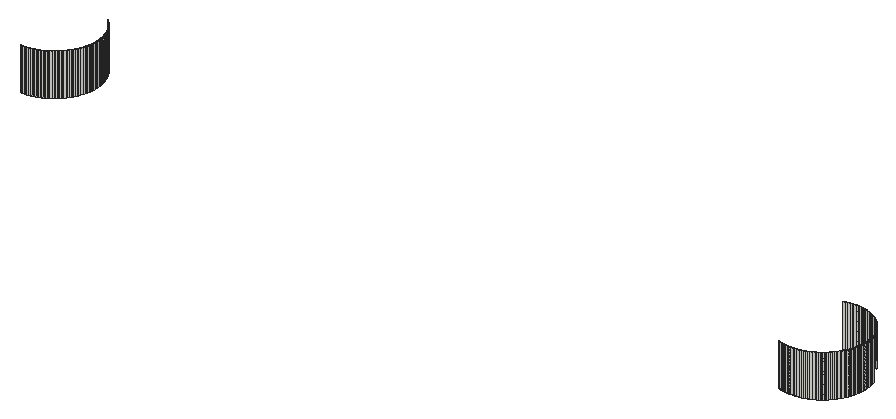
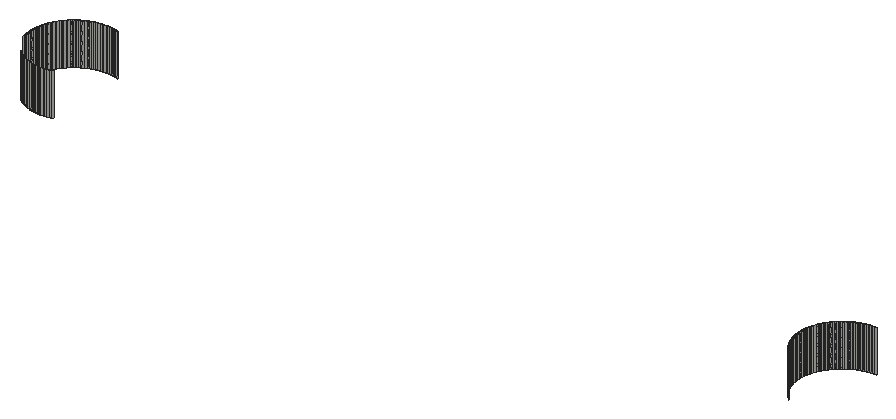
# SketchUp Ruby script. Lengths in inches.
U = 1.inch
M = Sketchup.active_model
def pt(a) = Geom::Point3d.new(a.map { |v| v * U })
def face(e, loops, mat)
  f = e.add_face(loops[0].map { |a| pt(a) })
  loops[1..].each { |l| e.add_face(l.map { |a| pt(a) }).erase! }
  f.material = f.back_material = mat if mat
  f
end
# faces: each face lists its corners as indices into pts; further lists are holes
def faces(e, pts, list, mat = nil) = list.each { |f| face(e, (f[0].is_a?(Array) ? f : [f]).map { |l| l.map { |i| pts[i] } }, mat) }
# xy, xz, yz: faces in a plane at the given z, y or x. An outline is a flat list of corners, or four numbers for a rectangle; further outlines are holes
def ring(l) = l.size == 4 ? [[l[0], l[1]], [l[2], l[1]], [l[2], l[3]], [l[0], l[3]]] : l.each_slice(2).to_a
def flat(e, list, mat, &to3) = list.each { |f| face(e, (f[0].is_a?(Array) ? f : [f]).map { |l| ring(l).map { |u, v| to3.(u, v) } }, mat) }
def xy(e, z, list, mat = nil) = flat(e, list, mat) { |x, y| [x, y, z] }
def xz(e, y, list, mat = nil) = flat(e, list, mat) { |x, z| [x, y, z] }
def yz(e, x, list, mat = nil) = flat(e, list, mat) { |y, z| [x, y, z] }
def lines(e, pts, list) = list.each { |a, b| e.add_line(pt(pts[a]), pt(pts[b])) }
# prism: a flat outline (further loops are holes) pulled along v
def prism(e, loops, v, mat = nil)
  f = face(e, loops, mat); d = Geom::Vector3d.new(v.map { |x| x * U })
  f.pushpull(f.normal.samedirection?(d) ? d.length : -d.length)
end
def box(e, o, s, mat = nil) = prism(e, [[o, [o[0] + s[0], o[1], o[2]], [o[0] + s[0], o[1] + s[1], o[2]], [o[0], o[1] + s[1], o[2]]]], [0, 0, s[2]], mat)
def at(x, y, z, deg = 0) = Geom::Transformation.translation(pt([x, y, z])) * Geom::Transformation.rotation(ORIGIN, Z_AXIS, deg.degrees)
def axes(o, x, y, z) = Geom::Transformation.new([*x, 0, *y, 0, *z, 0, *pt(o).to_a, 1])
def part(name) = M.definitions.add(name)
# library, detail: a bought-in or finely detailed component or shape, given as its bounding box
def library(name, o, s) = part(name).tap { |d| box(d.entities, o, s) }
def detail(e, o, s) = box(e.add_group.entities, o, s)
def put(e, d, t, mat = nil) = e.add_instance(d, t).tap { |i| i.material = mat if mat }
def group(e, t, mat = nil) = e.add_group.tap { |g| g.transformation = t; g.material = mat if mat }.entities
root = M.entities
xz(root,317,[[269.15,231,269.23,234],[269.23,231,269.3125,234],[323.875,231,323.95,234],[323.95,231,324.03,234],[324.03,231,324.11,234]])
xz(root,317.01,[[269.39,231,269.47,234],[323.72,231,323.8,234],[324.19,231,324.27,234]])
xz(root,322.99,[[323.73,231,323.81,234],[324.2,231,324.28,234]])
xz(root,323,[[323.89,231,323.97,234],[323.97,231,324.05,234],[324.05,231,324.125,234]])
yz(root,272.2,[[319.875,231,319.95,234],[319.95,231,320.03,234],[320.03,231,320.11,234]])
yz(root,326.99,[[319.72,231,319.8,234],[320.19,231,320.27,234]])
yz(root,327,[[319.875,231,319.95,234],[319.95,231,320.03,234],[320.03,231,320.11,234]])
p = [[269.39,317.01,231],[269.3125,317,231],[269.3125,317,234],[269.39,317.01,234],[269.625,317.03,231],[269.55,317.02,231],
  [269.55,317.02,234],[269.625,317.03,234],[269.47,317.01,231],[269.47,317.01,234],[269.7,317.04,231],[269.7,317.04,234],
  [269.78,317.06,231],[269.78,317.06,234],[323.49,317.04,231],[323.41,317.06,231],[323.41,317.06,234],[323.49,317.04,234],
  [323.5625,317.03,231],[323.5625,317.03,234],[323.72,317.01,231],[323.64,317.02,231],[323.64,317.02,234],[323.72,317.01,234],
  [323.875,317,231],[323.8,317.01,231],[323.8,317.01,234],[323.875,317,234],[324.19,317.01,231],[324.11,317,231],
  [324.11,317,234],[324.19,317.01,234],[324.42,317.03,231],[324.35,317.02,231],[324.35,317.02,234],[324.42,317.03,234],
  [324.27,317.01,231],[324.27,317.01,234],[324.5,317.04,231],[324.5,317.04,234],[324.58,317.06,231],[324.58,317.06,234],
  [269.86,317.07,231],[269.86,317.07,234],[270.01,317.11,231],[269.93,317.09,231],[269.93,317.09,234],[270.01,317.11,234],
  [270.08,317.13,231],[270.08,317.13,234],[270.16,317.16,231],[270.16,317.16,234],[323.18,317.11,231],[323.1,317.14,231],
  [323.1,317.14,234],[323.18,317.11,234],[323.26,317.09,231],[323.26,317.09,234],[323.33,317.08,231],[323.33,317.08,234],
  [324.66,317.07,231],[324.66,317.07,234],[324.81,317.11,231],[324.73,317.09,231],[324.73,317.09,234],[324.81,317.11,234],
  [324.88,317.13,231],[324.88,317.13,234],[324.96,317.16,231],[324.96,317.16,234],[270.31,317.21,231],[270.23,317.18,231],
  [270.23,317.18,234],[270.31,317.21,234],[270.38,317.24,231],[270.38,317.24,234],[270.45,317.27,231],[270.45,317.27,234],
  [325.11,317.21,231],[325.03,317.18,231],[325.03,317.18,234],[325.11,317.21,234],[325.18,317.24,231],[325.18,317.24,234],
  [325.25,317.27,231],[325.25,317.27,234],[270.59,317.34,231],[270.52,317.31,231],[270.52,317.31,234],[270.59,317.34,234],
  [270.66,317.38,231],[270.66,317.38,234],[325.39,317.34,231],[325.32,317.31,231],[325.32,317.31,234],[325.39,317.34,234],
  [325.46,317.38,231],[325.46,317.38,234],[270.8,317.46,231],[270.73,317.42,231],[270.73,317.42,234],[270.8,317.46,234],
  [325.6,317.46,231],[325.53,317.42,231],[325.53,317.42,234],[325.6,317.46,234],[270.86,317.5,231],[270.86,317.5,234],
  [270.99,317.59,231],[270.93,317.55,231],[270.93,317.55,234],[270.99,317.59,234],[325.66,317.5,231],[325.66,317.5,234],
  [325.79,317.59,231],[325.73,317.55,231],[325.73,317.55,234],[325.79,317.59,234],[271.05,317.64,231],[271.05,317.64,234],
  [271.11,317.69,231],[271.11,317.69,234],[325.85,317.64,231],[325.85,317.64,234],[325.91,317.69,231],[325.91,317.69,234],
  [271.17,317.74,231],[271.17,317.74,234],[271.23,317.79,231],[271.23,317.79,234],[325.97,317.74,231],[325.97,317.74,234],
  [326.03,317.79,231],[326.03,317.79,234],[271.29,317.85,231],[271.29,317.85,234],[271.34,317.9,231],[271.34,317.9,234],
  [326.09,317.85,231],[326.09,317.85,234],[326.14,317.9,231],[326.14,317.9,234],[271.4,317.96,231],[271.4,317.96,234],
  [326.2,317.96,231],[326.2,317.96,234],[271.45,318.02,231],[271.45,318.02,234],[271.5,318.08,231],[271.5,318.08,234],
  [326.25,318.02,231],[326.25,318.02,234],[326.3,318.08,231],[326.3,318.08,234],[271.55,318.14,231],[271.55,318.14,234],
  [271.6,318.2,231],[271.6,318.2,234],[326.35,318.14,231],[326.35,318.14,234],[326.4,318.2,231],[326.4,318.2,234],
  [271.65,318.26,231],[271.65,318.26,234],[326.45,318.26,231],[326.45,318.26,234],[271.69,318.33,231],[271.69,318.33,234],
  [271.73,318.39,231],[271.73,318.39,234],[326.49,318.33,231],[326.49,318.33,234],[326.53,318.39,231],[326.53,318.39,234],
  [271.78,318.46,231],[271.78,318.46,234],[326.58,318.46,231],[326.58,318.46,234],[271.85,318.6,231],[271.81,318.53,231],
  [271.81,318.53,234],[271.85,318.6,234],[326.65,318.6,231],[326.61,318.53,231],[326.61,318.53,234],[326.65,318.6,234],
  [271.89,318.67,231],[271.89,318.67,234],[326.6875,318.67,231],[326.6875,318.67,234],[271.95,318.81,231],[271.92,318.74,231],
  [271.92,318.74,234],[271.95,318.81,234],[326.75,318.81,231],[326.72,318.74,231],[326.72,318.74,234],[326.75,318.81,234],
  [271.98,318.88,231],[271.98,318.88,234],[326.78,318.88,231],[326.78,318.88,234],[272.01,318.96,231],[272.01,318.96,234],
  [326.8125,318.96,231],[326.8125,318.96,234],[272.0625,319.1,231],[272.04,319.03,231],[272.04,319.03,234],[272.0625,319.1,234],
  [326.86,319.1,231],[326.84,319.03,231],[326.84,319.03,234],[326.86,319.1,234],[272.09,319.18,231],[272.09,319.18,234],
  [326.89,319.18,231],[326.89,319.18,234],[272.11,319.26,231],[272.11,319.26,234],[326.91,319.26,231],[326.91,319.26,234],
  [272.14,319.41,231],[272.125,319.33,231],[272.125,319.33,234],[272.14,319.41,234],[326.94,319.41,231],[326.92,319.33,231],
  [326.92,319.33,234],[326.94,319.41,234],[272.16,319.49,231],[272.16,319.49,234],[326.96,319.49,231],[326.96,319.49,234],
  [272.17,319.5625,231],[272.17,319.5625,234],[326.97,319.5625,231],[326.97,319.5625,234],[272.1875,319.72,231],[272.18,319.64,231],
  [272.18,319.64,234],[272.1875,319.72,234],[326.99,319.72,231],[326.98,319.64,231],[326.98,319.64,234],[326.99,319.72,234],
  [272.19,319.8,231],[272.19,319.8,234],[272.2,319.875,231],[272.2,319.875,234],[327,319.875,231],[326.99,319.8,231],
  [326.99,319.8,234],[327,319.875,234],[272.19,320.19,231],[272.2,320.11,231],[272.2,320.11,234],[272.19,320.19,234],
  [326.99,320.19,231],[327,320.11,231],[327,320.11,234],[326.99,320.19,234],[272.1875,320.27,231],[272.1875,320.27,234],
  [272.17,320.42,231],[272.18,320.35,231],[272.18,320.35,234],[272.17,320.42,234],[326.97,320.42,231],[326.98,320.35,231],
  [326.98,320.35,234],[326.97,320.42,234],[326.99,320.27,231],[326.99,320.27,234],[272.16,320.5,231],[272.16,320.5,234],
  [326.96,320.5,231],[326.96,320.5,234],[272.14,320.58,231],[272.14,320.58,234],[326.94,320.58,231],[326.94,320.58,234],
  [272.13,320.66,231],[272.13,320.66,234],[326.93,320.66,231],[326.93,320.66,234],[272.09,320.81,231],[272.11,320.73,231],
  [272.11,320.73,234],[272.09,320.81,234],[326.89,320.81,231],[326.91,320.73,231],[326.91,320.73,234],[326.89,320.81,234],
  [272.07,320.88,231],[272.07,320.88,234],[326.87,320.88,231],[326.87,320.88,234],[272.04,320.96,231],[272.04,320.96,234],
  [271.99,321.11,231],[272.02,321.03,231],[272.02,321.03,234],[271.99,321.11,234],[271.96,321.18,231],[271.96,321.18,234],
  [271.93,321.25,231],[271.93,321.25,234],[271.86,321.39,231],[271.89,321.32,231],[271.89,321.32,234],[271.86,321.39,234],
  [271.82,321.46,231],[271.82,321.46,234],[271.74,321.6,231],[271.78,321.53,231],[271.78,321.53,234],[271.74,321.6,234],
  [271.7,321.66,231],[271.7,321.66,234],[271.61,321.79,231],[271.65,321.73,231],[271.65,321.73,234],[271.61,321.79,234],
  [271.56,321.85,231],[271.56,321.85,234],[271.46,321.97,231],[271.51,321.91,231],[271.51,321.91,234],[271.46,321.97,234],
  [271.35,322.09,231],[271.41,322.03,231],[271.41,322.03,234],[271.35,322.09,234],[271.24,322.2,231],[271.3,322.14,231],
  [271.3,322.14,234],[271.24,322.2,234],[271.18,322.25,231],[271.18,322.25,234],[325.86,322.35,231],[325.92,322.3,231],
  [325.92,322.3,234],[325.86,322.35,234],[325.98,322.25,231],[325.98,322.25,234],[325.67,322.49,231],[325.74,322.45,231],
  [325.74,322.45,234],[325.67,322.49,234],[325.8,322.4,231],[325.8,322.4,234],[325.54,322.58,231],[325.61,322.53,231],
  [325.61,322.53,234],[325.54,322.58,234],[325.4,322.65,231],[325.47,322.61,231],[325.47,322.61,234],[325.4,322.65,234],
  [325.19,322.75,231],[325.26,322.72,231],[325.26,322.72,234],[325.19,322.75,234],[325.33,322.6875,231],[325.33,322.6875,234],
  [324.9,322.86,231],[324.97,322.84,231],[324.97,322.84,234],[324.9,322.86,234],[325.04,322.8125,231],[325.04,322.8125,234],
  [325.12,322.78,231],[325.12,322.78,234],[323.12,322.87,231],[323.19,322.89,231],[323.19,322.89,234],[323.12,322.87,234],
  [323.27,322.91,231],[323.27,322.91,234],[323.34,322.93,231],[323.34,322.93,234],[323.42,322.94,231],[323.42,322.94,234],
  [323.5,322.96,231],[323.5,322.96,234],[324.51,322.96,231],[324.59,322.94,231],[324.59,322.94,234],[324.51,322.96,234],
  [324.67,322.92,231],[324.67,322.92,234],[324.74,322.91,231],[324.74,322.91,234],[324.82,322.89,231],[324.82,322.89,234],
  [323.58,322.97,231],[323.58,322.97,234],[323.65,322.98,231],[323.65,322.98,234],[323.73,322.99,231],[323.73,322.99,234],
  [323.81,322.99,231],[323.89,323,231],[323.89,323,234],[323.81,322.99,234],[324.125,323,231],[324.2,322.99,231],
  [324.2,322.99,234],[324.125,323,234],[324.28,322.99,231],[324.36,322.98,231],[324.36,322.98,234],[324.28,322.99,234],
  [324.4375,322.97,231],[324.4375,322.97,234]]
faces(root,p,[[0,1,2,3],[4,5,6,7],[5,8,9,6],[10,4,7,11],[12,10,11,13],[14,15,16,17],[18,14,17,19],[20,21,22,23],
  [21,18,19,22],[24,25,26,27],[28,29,30,31],[32,33,34,35],[33,36,37,34],[38,32,35,39],[40,38,39,41],[42,12,13,43],
  [44,45,46,47],[45,42,43,46],[48,44,47,49],[50,48,49,51],[52,53,54,55],[56,52,55,57],[15,58,59,16],[58,56,57,59],
  [60,40,41,61],[62,63,64,65],[63,60,61,64],[66,62,65,67],[68,66,67,69],[70,71,72,73],[71,50,51,72],[74,70,73,75],
  [76,74,75,77],[78,79,80,81],[79,68,69,80],[82,78,81,83],[84,82,83,85],[86,87,88,89],[87,76,77,88],[90,86,89,91],
  [92,93,94,95],[93,84,85,94],[96,92,95,97],[98,99,100,101],[99,90,91,100],[102,103,104,105],[103,96,97,104],[106,98,101,107],
  [108,109,110,111],[109,106,107,110],[112,102,105,113],[114,115,116,117],[115,112,113,116],[118,108,111,119],[120,118,119,121],[122,114,117,123],
  [124,122,123,125],[126,120,121,127],[128,126,127,129],[130,124,125,131],[132,130,131,133],[134,128,129,135],[136,134,135,137],[138,132,133,139],
  [140,138,139,141],[142,136,137,143],[144,140,141,145],[146,142,143,147],[148,146,147,149],[150,144,145,151],[152,150,151,153],[154,148,149,155],
  [156,154,155,157],[158,152,153,159],[160,158,159,161],[162,156,157,163],[164,160,161,165],[166,162,163,167],[168,166,167,169],[170,164,165,171],
  [172,170,171,173],[174,168,169,175],[176,172,173,177],[178,179,180,181],[179,174,175,180],[182,183,184,185],[183,176,177,184],[186,178,181,187],
  [188,182,185,189],[190,191,192,193],[191,186,187,192],[194,195,196,197],[195,188,189,196],[198,190,193,199],[200,194,197,201],[202,198,199,203],
  [204,200,201,205],[206,207,208,209],[207,202,203,208],[210,211,212,213],[211,204,205,212],[214,206,209,215],[216,210,213,217],[218,214,215,219],
  [220,216,217,221],[222,223,224,225],[223,218,219,224],[226,227,228,229],[227,220,221,228],[230,222,225,231],[232,226,229,233],[234,230,231,235],
  [236,232,233,237],[238,239,240,241],[239,234,235,240],[242,243,244,245],[243,236,237,244],[246,238,241,247],[248,246,247,249],[250,251,252,253],
  [254,255,256,257],[258,259,260,261],[262,254,257,263],[264,265,266,267],[265,262,263,266],[268,269,270,271],[269,272,273,270],[274,264,267,275],
  [276,268,271,277],[278,274,275,279],[280,276,277,281],[282,278,279,283],[284,280,281,285],[286,287,288,289],[287,282,283,288],[290,291,292,293],
  [291,284,285,292],[294,286,289,295],[296,290,293,297],[298,294,295,299],[300,301,302,303],[301,298,299,302],[304,300,303,305],[306,304,305,307],
  [308,309,310,311],[309,306,307,310],[312,308,311,313],[314,315,316,317],[315,312,313,316],[318,314,317,319],[320,321,322,323],[321,318,319,322],
  [324,320,323,325],[326,327,328,329],[327,324,325,328],[330,331,332,333],[331,326,329,332],[334,335,336,337],[335,330,333,336],[338,334,337,339],
  [340,341,342,343],[341,344,345,342],[346,347,348,349],[347,350,351,348],[350,340,343,351],[352,353,354,355],[353,346,349,354],[356,357,358,359],
  [357,352,355,358],[360,361,362,363],[361,364,365,362],[364,356,359,365],[366,367,368,369],[367,370,371,368],[370,372,373,371],[372,360,363,373],
  [374,375,376,377],[375,378,379,376],[378,380,381,379],[380,382,383,381],[382,384,385,383],[386,387,388,389],[387,390,391,388],[390,392,393,391],
  [392,394,395,393],[394,366,369,395],[384,396,397,385],[396,398,399,397],[398,400,401,399],[402,403,404,405],[406,407,408,409],[410,411,412,413],
  [411,414,415,412],[414,386,389,415]])
